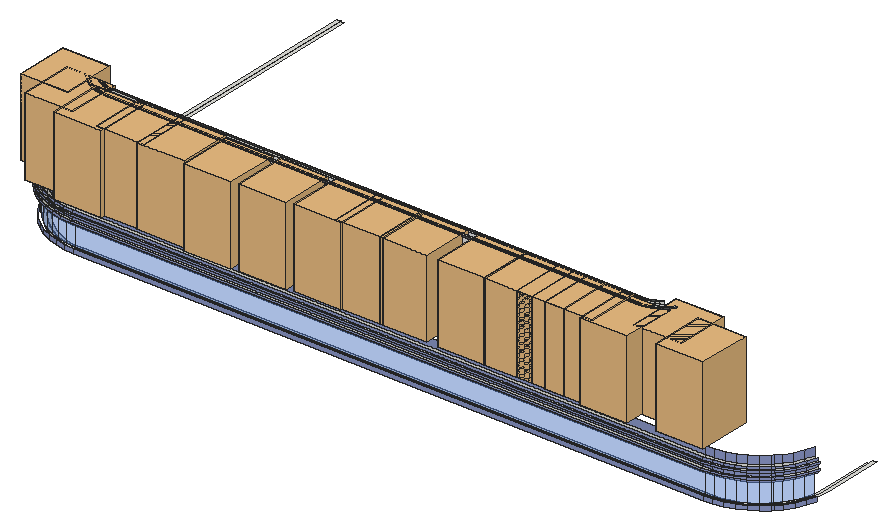
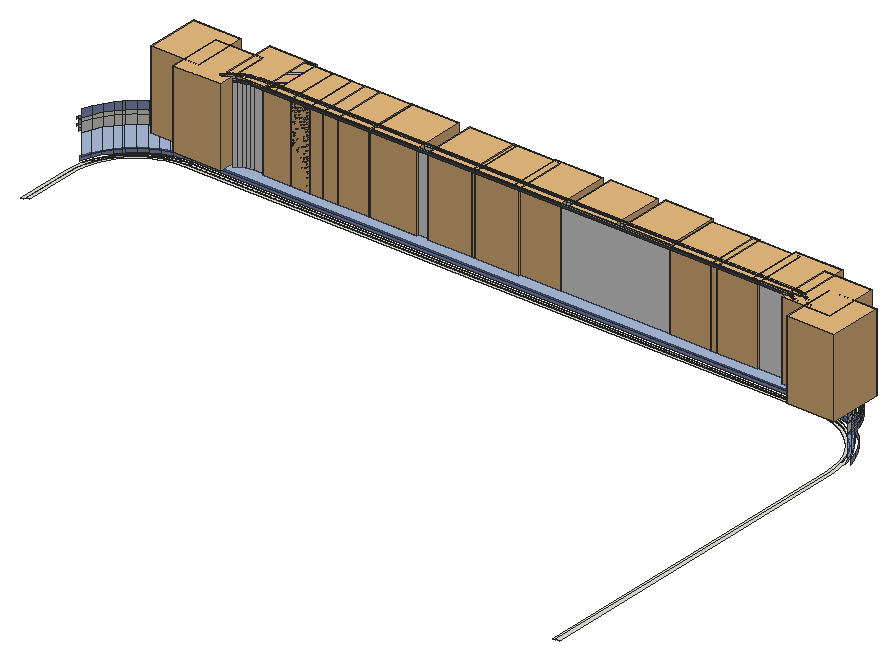
# SketchUp Ruby script. Lengths in inches.
U = 1.inch
M = Sketchup.active_model
def pt(a) = Geom::Point3d.new(a.map { |v| v * U })
def face(e, loops, mat)
  f = e.add_face(loops[0].map { |a| pt(a) })
  loops[1..].each { |l| e.add_face(l.map { |a| pt(a) }).erase! }
  f.material = f.back_material = mat if mat
  f
end
# faces: each face lists its corners as indices into pts; further lists are holes
def faces(e, pts, list, mat = nil) = list.each { |f| face(e, (f[0].is_a?(Array) ? f : [f]).map { |l| l.map { |i| pts[i] } }, mat) }
# xy, xz, yz: faces in a plane at the given z, y or x. An outline is a flat list of corners, or four numbers for a rectangle; further outlines are holes
def ring(l) = l.size == 4 ? [[l[0], l[1]], [l[2], l[1]], [l[2], l[3]], [l[0], l[3]]] : l.each_slice(2).to_a
def flat(e, list, mat, &to3) = list.each { |f| face(e, (f[0].is_a?(Array) ? f : [f]).map { |l| ring(l).map { |u, v| to3.(u, v) } }, mat) }
def xy(e, z, list, mat = nil) = flat(e, list, mat) { |x, y| [x, y, z] }
def xz(e, y, list, mat = nil) = flat(e, list, mat) { |x, z| [x, y, z] }
def yz(e, x, list, mat = nil) = flat(e, list, mat) { |y, z| [x, y, z] }
def lines(e, pts, list) = list.each { |a, b| e.add_line(pt(pts[a]), pt(pts[b])) }
# prism: a flat outline (further loops are holes) pulled along v
def prism(e, loops, v, mat = nil)
  f = face(e, loops, mat); d = Geom::Vector3d.new(v.map { |x| x * U })
  f.pushpull(f.normal.samedirection?(d) ? d.length : -d.length)
end
def box(e, o, s, mat = nil) = prism(e, [[o, [o[0] + s[0], o[1], o[2]], [o[0] + s[0], o[1] + s[1], o[2]], [o[0], o[1] + s[1], o[2]]]], [0, 0, s[2]], mat)
def at(x, y, z, deg = 0) = Geom::Transformation.translation(pt([x, y, z])) * Geom::Transformation.rotation(ORIGIN, Z_AXIS, deg.degrees)
def axes(o, x, y, z) = Geom::Transformation.new([*x, 0, *y, 0, *z, 0, *pt(o).to_a, 1])
def part(name) = M.definitions.add(name)
# library, detail: a bought-in or finely detailed component or shape, given as its bounding box
def library(name, o, s) = part(name).tap { |d| box(d.entities, o, s) }
def detail(e, o, s) = box(e.add_group.entities, o, s)
def put(e, d, t, mat = nil) = e.add_instance(d, t).tap { |i| i.material = mat if mat }
def group(e, t, mat = nil) = e.add_group.tap { |g| g.transformation = t; g.material = mat if mat }.entities
root = M.entities
M.materials.add("0326 AP 7207 CLASSIC PURPLE").color = [140, 152, 201]
M.materials.add("[Color M06]").color = [86, 86, 86]
M.materials.add("[Mirror 02]").color = [229, 229, 229]
M.materials.add("[Translucent Glass Blue]").color = [100, 149, 237]
M.materials["[Translucent Glass Blue]"].alpha = 0.5
c1 = library("Ficus elastica Belize 002",[-7.92,-8.8125,0.01],[22.14,24.73,36.43])
xy(root,252.375,[[45.79,28.41,41.61,28.68,37.51,29.49,33.55,30.84,29.8,32.6875,26.32,35.01,23.18,37.77,20.42,40.91,18.1,44.39,16.25,48.14,14.9,52.1,14.09,56.21,13.8125,60.38,13.8125,220.92,15.26,220.92,15.26,60.38,15.53,56.4,16.3,52.48,17.59,48.7,19.35,45.12,21.57,41.8,24.2,38.8,27.21,36.16,30.53,33.95,34.11,32.18,37.89,30.9,41.8,30.12,45.79,29.86,340.48,29.86,344.41,30.12,348.15,30.86,351.77,32.09,355.19,33.78,358.37,35.9,361.24,38.42,361.69,38.9375,363.76,41.29,365.88,44.46,367.57,47.89,368.8,51.51,369.54,55.25,369.8,59.18,369.8,84.09,371.25,84.09,371.25,59.13,370.98,55.0625,370.2,51.13,368.91,47.33,367.14,43.74,364.91,40.4,362.79,37.98,362.27,37.39,359.25,34.74,355.92,32.52,352.32,30.74,348.53,29.45,344.6,28.67,340.52,28.41]])
xy(root,252.5625,[[45.79,26.99,41.43,27.28,37.15,28.13,33.01,29.54,29.09,31.47,25.46,33.89,22.18,36.77,19.3,40.06,16.875,43.6875,14.94,47.6,13.54,51.74,12.6875,56.02,12.4,60.38,12.4,220.92,13.8125,220.92,13.8125,60.38,14.09,56.21,14.9,52.1,16.25,48.14,18.1,44.39,20.42,40.91,23.18,37.77,26.32,35.01,29.8,32.6875,33.55,30.84,37.51,29.49,41.61,28.68,45.79,28.41,340.52,28.41,344.6,28.67,348.53,29.45,352.32,30.74,355.92,32.52,359.25,34.74,362.27,37.39,362.79,37.98,364.91,40.4,367.14,43.74,368.91,47.33,370.2,51.13,370.98,55.0625,371.25,59.13,371.25,86.25,372.66,86.25,372.66,59.09,372.39,54.88,371.57,50.76,370.22,46.79,368.36,43.03,366.03,39.54,363.85,37.05,363.27,36.39,360.11,33.62,356.63,31.29,352.87,29.4375,348.89,28.09,344.78,27.27,340.57,26.99]])
xz(root,23.28,[[45.79,265.875,340.69,266.8125],[45.79,268.875,340.69,269.625]],"0326 AP 7207 CLASSIC PURPLE")
xz(root,24.43,[[45.79,265.875,340.65,266.8125],[45.79,268.875,340.65,269.625]])
xz(root,24.43,[[45.79,264.4375,340.65,265.875],[45.79,266.8125,340.65,268.875],[45.79,269.625,340.65,270.75]],"0326 AP 7207 CLASSIC PURPLE")
xz(root,24.97,[[45.79,252,340.64,254.0625]],"0326 AP 7207 CLASSIC PURPLE")
xz(root,26.25,[[45.79,264.4375,340.59,268.875],[45.79,268.875,340.59,270.75]])
xz(root,26.25,[[45.79,270.75,340.59,274.4375]],"0326 AP 7207 CLASSIC PURPLE")
xz(root,26.25,[[45.79,254.0625,340.59,264.4375]],"[Translucent Glass Blue]")
xz(root,26.99,[[45.79,252,340.57,252.5625]])
xz(root,28.41,[[45.79,252,340.52,252.375],[45.79,252.375,340.52,252.5625]])
xz(root,42.77,[[45.79,310.4375,294.9,311.125]],"[Color M06]")
xz(root,43.83,[[45.79,310.4375,294.87,311.125]])
xz(root,43.83,[[45.79,274.4375,294.87,310.4375]],"[Mirror 02]")
xz(root,47,[[45.79,310.4375,294.72,311.125]])
xz(root,47,[[45.79,274.4375,294.72,310.4375]],"[Mirror 02]")
xz(root,48.0625,[[45.79,310.4375,294.72,311.125]],"[Color M06]")
p = [[41.16,25.28,252],[45.79,24.97,252],[45.79,24.97,254.0625],[41.16,25.28,254.0625],[340.64,24.97,252],[345.04,25.26,252],
  [345.04,25.26,254.0625],[340.64,24.97,254.0625],[36.62,26.18,252],[36.62,26.18,254.0625],[349.42,26.13,252],[349.42,26.13,254.0625],
  [353.64,27.57,252],[353.64,27.57,254.0625],[32.24,27.67,252],[32.24,27.67,254.0625],[45.79,26.99,252],[41.43,27.28,252],
  [41.43,27.28,252.5625],[45.79,26.99,252.5625],[344.78,27.27,252],[340.57,26.99,252],[340.57,26.99,252.5625],[344.78,27.27,252.5625],
  [37.15,28.13,252],[37.15,28.13,252.5625],[348.89,28.09,252],[348.89,28.09,252.5625],[357.64,29.54,252],[357.64,29.54,254.0625],
  [28.08,29.72,252],[28.08,29.72,254.0625],[33.01,29.54,252],[33.01,29.54,252.5625],[352.87,29.4375,252],[352.87,29.4375,252.5625],
  [41.61,28.68,252],[45.79,28.41,252],[45.79,28.41,252.375],[41.61,28.68,252.375],[340.52,28.41,252],[344.6,28.67,252],
  [344.6,28.67,252.375],[340.52,28.41,252.375],[37.51,29.49,252],[37.51,29.49,252.375],[348.53,29.45,252],[348.53,29.45,252.375],
  [356.63,31.29,252],[356.63,31.29,252.5625],[29.09,31.47,252],[29.09,31.47,252.5625],[33.55,30.84,252],[33.55,30.84,252.375],
  [352.32,30.74,252],[352.32,30.74,252.375],[361.35,32.02,252],[361.35,32.02,254.0625],[24.23,32.29,252],[24.23,32.29,254.0625],
  [355.92,32.52,252],[355.92,32.52,252.375],[29.8,32.6875,252],[29.8,32.6875,252.375],[360.11,33.62,252],[360.11,33.62,252.5625],
  [25.46,33.89,252],[25.46,33.89,252.5625],[364.7,34.96,252],[364.7,34.96,254.0625],[20.75,35.34,252],[20.75,35.34,254.0625],
  [359.25,34.74,252],[359.25,34.74,252.375],[26.32,35.01,252],[26.32,35.01,252.375],[363.27,36.39,252],[363.27,36.39,252.5625],
  [22.18,36.77,252],[22.18,36.77,252.5625],[362.27,37.39,252],[362.27,37.39,252.375],[23.18,37.77,252],[23.18,37.77,252.375],
  [365.37,35.72,252],[365.37,35.72,254.0625],[17.7,38.83,252],[17.7,38.83,254.0625],[367.64,38.31,252],[367.64,38.31,254.0625],
  [363.85,37.05,252],[363.85,37.05,252.5625],[19.3,40.06,252],[19.3,40.06,252.5625],[366.03,39.54,252],[366.03,39.54,252.5625],
  [362.79,37.98,252],[362.79,37.98,252.375],[20.42,40.91,252],[20.42,40.91,252.375],[364.91,40.4,252],[364.91,40.4,252.375],
  [370.12,42.02,252],[370.12,42.02,254.0625],[15.125,42.68,252],[15.125,42.68,254.0625],[368.36,43.03,252],[368.36,43.03,252.5625],
  [16.875,43.6875,252],[16.875,43.6875,252.5625],[367.14,43.74,252],[367.14,43.74,252.375],[18.1,44.39,252],[18.1,44.39,252.375],
  [372.09,46.02,252],[372.09,46.02,254.0625],[13.08,46.83,252],[13.08,46.83,254.0625],[370.22,46.79,252],[370.22,46.79,252.5625],
  [14.94,47.6,252],[14.94,47.6,252.5625],[368.91,47.33,252],[368.91,47.33,252.375],[16.25,48.14,252],[16.25,48.14,252.375],
  [373.52,50.24,252],[373.52,50.24,254.0625],[11.59,51.22,252],[11.59,51.22,254.0625],[371.57,50.76,252],[371.57,50.76,252.5625],
  [370.2,51.13,252],[370.2,51.13,252.375],[13.54,51.74,252],[13.54,51.74,252.5625],[14.9,52.1,252],[14.9,52.1,252.375],
  [41.61,28.68,252.5625],[45.79,28.41,252.5625],[340.52,28.41,252.5625],[344.6,28.67,252.5625],[37.51,29.49,252.5625],[348.53,29.45,252.5625],
  [33.55,30.84,252.5625],[352.32,30.74,252.5625],[355.92,32.52,252.5625],[29.8,32.6875,252.5625],[359.25,34.74,252.5625],[26.32,35.01,252.5625],
  [362.27,37.39,252.5625],[23.18,37.77,252.5625],[362.79,37.98,252.5625],[20.42,40.91,252.5625],[364.91,40.4,252.5625],[367.14,43.74,252.5625],
  [18.1,44.39,252.5625],[368.91,47.33,252.5625],[16.25,48.14,252.5625],[370.2,51.13,252.5625],[14.9,52.1,252.5625],[45.79,26.25,254.0625],
  [45.79,26.25,264.4375],[41.33,26.54,264.4375],[41.33,26.54,254.0625],[344.88,26.53,254.0625],[344.88,26.53,264.4375],[340.59,26.25,264.4375],
  [340.59,26.25,254.0625],[36.95,27.41,264.4375],[36.95,27.41,254.0625],[349.09,27.37,254.0625],[349.09,27.37,264.4375],[32.73,28.85,264.4375],
  [32.73,28.85,254.0625],[353.15,28.75,254.0625],[353.15,28.75,264.4375],[357,30.65,254.0625],[357,30.65,264.4375],[28.72,30.82,264.4375],
  [28.72,30.82,254.0625],[360.57,33.03,254.0625],[360.57,33.03,264.4375],[25.01,33.3,264.4375],[25.01,33.3,254.0625],[363.8,35.86,254.0625],
  [363.8,35.86,264.4375],[21.65,36.25,264.4375],[21.65,36.25,254.0625],[364.41,36.56,254.0625],[364.41,36.56,264.4375],[18.71,39.6,264.4375],
  [18.71,39.6,254.0625],[366.625,39.09,254.0625],[366.625,39.09,264.4375],[369.01,42.66,254.0625],[369.01,42.66,264.4375],[16.23,43.31,264.4375],
  [16.23,43.31,254.0625],[370.91,46.51,254.0625],[370.91,46.51,264.4375],[14.25,47.32,264.4375],[14.25,47.32,254.0625],[372.29,50.57,254.0625],
  [372.29,50.57,264.4375],[12.82,51.55,264.4375],[12.82,51.55,254.0625],[45.79,24.43,265.875],[41.09,24.74,265.875],[41.09,24.74,264.4375],
  [45.79,24.43,264.4375],[345.11,24.73,265.875],[340.65,24.43,265.875],[340.65,24.43,264.4375],[345.11,24.73,264.4375],[36.48,25.66,265.875],
  [36.48,25.66,264.4375],[349.56,25.61,265.875],[349.56,25.61,264.4375],[353.85,27.07,265.875],[353.85,27.07,264.4375],[32.03,27.17,265.875],
  [32.03,27.17,264.4375],[45.79,26.25,268.875],[41.33,26.54,268.875],[344.88,26.53,268.875],[340.59,26.25,268.875],[36.95,27.41,268.875],
  [349.09,27.37,268.875],[357.91,29.07,265.875],[357.91,29.07,264.4375],[27.8125,29.25,265.875],[27.8125,29.25,264.4375],[32.73,28.85,268.875],
  [353.15,28.75,268.875],[357,30.65,268.875],[28.72,30.82,268.875],[361.68,31.59,265.875],[361.68,31.59,264.4375],[23.9,31.86,265.875],
  [23.9,31.86,264.4375],[360.57,33.03,268.875],[25.01,33.3,268.875],[365.08,34.57,265.875],[365.08,34.57,264.4375],[20.37,34.96,265.875],
  [20.37,34.96,264.4375],[363.8,35.86,268.875],[21.65,36.25,268.875],[365.77,35.36,265.875],[365.77,35.36,264.4375],[17.27,38.5,265.875],
  [17.27,38.5,264.4375],[368.07,37.98,265.875],[368.07,37.98,264.4375],[364.41,36.56,268.875],[18.71,39.6,268.875],[366.625,39.09,268.875],
  [370.59,41.75,265.875],[370.59,41.75,264.4375],[14.66,42.41,265.875],[14.66,42.41,264.4375],[369.01,42.66,268.875],[16.23,43.31,268.875],
  [372.59,45.81,265.875],[372.59,45.81,264.4375],[12.58,46.625,265.875],[12.58,46.625,264.4375],[370.91,46.51,268.875],[14.25,47.32,268.875],
  [374.05,50.1,265.875],[374.05,50.1,264.4375],[372.29,50.57,268.875],[11.07,51.08,265.875],[11.07,51.08,264.4375],[12.82,51.55,268.875],
  [40.94,23.6,265.875],[45.79,23.28,265.875],[45.79,23.28,266.8125],[40.94,23.6,266.8125],[340.69,23.28,265.875],[345.27,23.58,265.875],
  [345.27,23.58,266.8125],[340.69,23.28,266.8125],[36.18,24.54,265.875],[36.18,24.54,266.8125],[349.86,24.49,265.875],[349.86,24.49,266.8125],
  [45.79,24.43,266.8125],[41.09,24.74,266.8125],[345.11,24.73,266.8125],[340.65,24.43,266.8125],[31.59,26.1,265.875],[31.59,26.1,266.8125],
  [354.29,26,265.875],[354.29,26,266.8125],[36.48,25.66,266.8125],[349.56,25.61,266.8125],[353.85,27.07,266.8125],[32.03,27.17,266.8125],
  [358.49,28.07,265.875],[358.49,28.07,266.8125],[27.24,28.25,265.875],[27.24,28.25,266.8125],[357.91,29.07,266.8125],[27.8125,29.25,266.8125],
  [362.38,30.67,265.875],[362.38,30.67,266.8125],[23.2,30.95,265.875],[23.2,30.95,266.8125],[361.68,31.59,266.8125],[23.9,31.86,266.8125],
  [365.9,33.76,265.875],[365.9,33.76,266.8125],[19.55,34.15,265.875],[19.55,34.15,266.8125],[365.08,34.57,266.8125],[20.37,34.96,266.8125],
  [366.64,34.6,265.875],[366.64,34.6,266.8125],[16.35,37.8,265.875],[16.35,37.8,266.8125],[365.77,35.36,266.8125],[368.99,37.28,265.875],
  [368.99,37.28,266.8125],[17.27,38.5,266.8125],[368.07,37.98,266.8125],[371.59,41.17,265.875],[371.59,41.17,266.8125],[13.66,41.83,265.875],
  [13.66,41.83,266.8125],[370.59,41.75,266.8125],[14.66,42.41,266.8125],[373.66,45.37,265.875],[373.66,45.37,266.8125],[372.59,45.81,266.8125],
  [11.51,46.18,265.875],[11.51,46.18,266.8125],[12.58,46.625,266.8125],[375.16,49.8,265.875],[375.16,49.8,266.8125],[374.05,50.1,266.8125],
  [9.95,50.78,265.875],[9.95,50.78,266.8125],[11.07,51.08,266.8125],[41.09,24.74,268.875],[45.79,24.43,268.875],[340.65,24.43,268.875],
  [345.11,24.73,268.875],[36.48,25.66,268.875],[349.56,25.61,268.875],[353.85,27.07,268.875],[32.03,27.17,268.875],[357.91,29.07,268.875],
  [27.8125,29.25,268.875],[361.68,31.59,268.875],[23.9,31.86,268.875],[365.08,34.57,268.875],[20.37,34.96,268.875],[365.77,35.36,268.875],
  [17.27,38.5,268.875],[368.07,37.98,268.875],[370.59,41.75,268.875],[14.66,42.41,268.875],[372.59,45.81,268.875],[12.58,46.625,268.875],
  [374.05,50.1,268.875],[11.07,51.08,268.875],[40.94,23.6,268.875],[45.79,23.28,268.875],[45.79,23.28,269.625],[40.94,23.6,269.625],
  [340.69,23.28,268.875],[345.27,23.58,268.875],[345.27,23.58,269.625],[340.69,23.28,269.625],[36.18,24.55,268.875],[36.18,24.55,269.625],
  [349.86,24.5,268.875],[349.86,24.5,269.625],[45.79,24.43,269.625],[41.09,24.74,269.625],[345.11,24.73,269.625],[340.65,24.43,269.625],
  [31.59,26.11,268.875],[31.59,26.11,269.625],[354.29,26,268.875],[354.29,26,269.625],[36.48,25.66,269.625],[349.56,25.61,269.625],
  [353.85,27.07,269.625],[32.03,27.17,269.625],[358.49,28.07,268.875],[358.49,28.07,269.625],[27.24,28.25,268.875],[27.24,28.25,269.625],
  [45.79,26.25,270.75],[41.33,26.54,270.75],[344.88,26.53,270.75],[340.59,26.25,270.75],[36.95,27.41,270.75],[349.09,27.37,270.75],
  [357.91,29.07,269.625],[27.8125,29.25,269.625],[32.73,28.85,270.75],[353.15,28.75,270.75],[362.38,30.67,268.875],[362.38,30.67,269.625],
  [23.2,30.95,268.875],[23.2,30.95,269.625],[357,30.65,270.75],[28.72,30.82,270.75],[361.68,31.59,269.625],[23.9,31.86,269.625],
  [360.57,33.03,270.75],[365.9,33.76,268.875],[365.9,33.76,269.625],[25.01,33.3,270.75],[19.56,34.15,268.875],[19.56,34.15,269.625],
  [365.08,34.57,269.625],[20.37,34.96,269.625],[363.8,35.86,270.75],[21.65,36.25,270.75],[366.64,34.6,268.875],[366.64,34.6,269.625],
  [16.36,37.8,268.875],[16.36,37.8,269.625],[365.77,35.36,269.625],[368.98,37.28,268.875],[368.98,37.28,269.625],[17.27,38.5,269.625],
  [368.07,37.98,269.625],[364.41,36.56,270.75],[18.71,39.6,270.75],[366.625,39.09,270.75],[371.59,41.17,268.875],[371.59,41.17,269.625],
  [13.66,41.83,268.875],[13.66,41.83,269.625],[370.59,41.75,269.625],[14.66,42.41,269.625],[369.01,42.66,270.75],[16.23,43.31,270.75],
  [373.66,45.37,268.875],[373.66,45.37,269.625],[372.59,45.81,269.625],[11.51,46.18,268.875],[11.51,46.18,269.625],[12.58,46.625,269.625],
  [370.91,46.51,270.75],[14.25,47.32,270.75],[375.16,49.8,268.875],[375.16,49.8,269.625],[374.05,50.1,269.625],[9.95,50.78,268.875],
  [9.95,50.78,269.625],[372.29,50.57,270.75],[11.07,51.08,269.625],[12.82,51.55,270.75],[41.09,24.74,270.75],[45.79,24.43,270.75],
  [340.65,24.43,270.75],[345.11,24.73,270.75],[36.48,25.66,270.75],[349.56,25.61,270.75],[353.85,27.07,270.75],[32.03,27.17,270.75],
  [357.91,29.07,270.75],[27.8125,29.25,270.75],[361.68,31.59,270.75],[23.9,31.86,270.75],[365.08,34.57,270.75],[20.37,34.96,270.75],
  [365.77,35.36,270.75],[17.27,38.5,270.75],[368.07,37.98,270.75],[370.59,41.75,270.75],[14.66,42.41,270.75],[372.59,45.81,270.75],
  [12.58,46.625,270.75],[374.05,50.1,270.75],[11.07,51.08,270.75],[45.79,26.25,274.4375],[41.33,26.54,274.4375],[344.88,26.53,274.4375],
  [340.59,26.25,274.4375],[36.95,27.41,274.4375],[349.09,27.37,274.4375],[32.73,28.85,274.4375],[353.15,28.75,274.4375],[357,30.65,274.4375],
  [28.72,30.82,274.4375],[360.57,33.03,274.4375],[25.01,33.3,274.4375],[363.8,35.86,274.4375],[21.65,36.25,274.4375],[364.41,36.56,274.4375],
  [18.71,39.6,274.4375],[366.625,39.09,274.4375],[369.01,42.66,274.4375],[16.23,43.31,274.4375],[370.91,46.51,274.4375],[14.25,47.32,274.4375],
  [372.29,50.57,274.4375],[12.82,51.55,274.4375],[43.625,43.97,274.4375],[45.79,43.83,274.4375],[45.79,43.83,310.4375],[43.625,43.97,310.4375],
  [294.87,43.83,274.4375],[296.8,43.96,274.4375],[296.8,43.96,310.4375],[294.87,43.83,310.4375],[41.5,44.4,274.4375],[41.5,44.4,310.4375],
  [298.85,44.37,274.4375],[298.85,44.37,310.4375],[39.45,45.09,274.4375],[39.45,45.09,310.4375],[300.82,45.04,274.4375],[300.82,45.04,310.4375],
  [302.69,45.96,274.4375],[302.69,45.96,310.4375],[37.51,46.05,274.4375],[37.51,46.05,310.4375],[35.71,47.25,274.4375],[35.71,47.25,310.4375],
  [304.25,47,274.4375],[304.25,47,310.4375],[45.79,47,274.4375],[44.04,47.11,274.4375],[44.04,47.11,310.4375],[45.79,47,310.4375],
  [296.39,47.11,274.4375],[294.72,47,274.4375],[294.72,47,310.4375],[296.39,47.11,310.4375],[304.43,47.12,274.4375],[304.43,47.12,310.4375],
  [42.32,47.45,274.4375],[42.32,47.45,310.4375],[298.03,47.43,274.4375],[298.03,47.43,310.4375],[306,48.49,274.4375],[306,48.49,310.4375],
  [34.09,48.68,274.4375],[34.09,48.68,310.4375],[299.61,47.97,274.4375],[299.61,47.97,310.4375],[40.67,48.02,274.4375],[40.67,48.02,310.4375],
  [39.1,48.79,274.4375],[39.1,48.79,310.4375],[301.11,48.71,274.4375],[301.11,48.71,310.4375],[307.375,50.0625,274.4375],[307.375,50.0625,310.4375],
  [32.66,50.31,274.4375],[32.66,50.31,310.4375],[302.5,49.64,274.4375],[302.5,49.64,310.4375],[37.64,49.76,274.4375],[37.64,49.76,310.4375],
  [307.49,50.24,274.4375],[307.49,50.24,310.4375],[43.49,42.92,310.4375],[45.79,42.77,310.4375],[45.79,42.77,311.125],[43.49,42.92,311.125],
  [294.9,42.77,310.4375],[296.94,42.9,310.4375],[296.94,42.9,311.125],[294.9,42.77,311.125],[41.23,43.37,310.4375],[41.23,43.37,311.125],
  [299.125,43.34,310.4375],[299.125,43.34,311.125],[301.23,44.05,310.4375],[301.23,44.05,311.125],[39.05,44.11,310.4375],[39.05,44.11,311.125],
  [43.625,43.97,311.125],[45.79,43.83,311.125],[294.87,43.83,311.125],[296.8,43.96,311.125],[41.5,44.4,311.125],[298.85,44.37,311.125],
  [36.98,45.13,310.4375],[36.98,45.13,311.125],[303.23,45.04,310.4375],[303.23,45.04,311.125],[39.45,45.09,311.125],[300.82,45.04,311.125],
  [302.69,45.96,311.125],[304.84,46.11,310.4375],[304.84,46.11,311.125],[35.07,46.41,310.4375],[35.07,46.41,311.125],[37.51,46.05,311.125],
  [35.71,47.25,311.125],[304.25,47,311.125],[305.08,46.27,310.4375],[305.08,46.27,311.125],[306.75,47.74,310.4375],[306.75,47.74,311.125],
  [33.33,47.93,310.4375],[33.33,47.93,311.125],[45.79,47,311.125],[44.04,47.11,311.125],[296.39,47.11,311.125],[294.72,47,311.125],
  [304.43,47.12,311.125],[42.32,47.45,311.125],[298.03,47.43,311.125],[306,48.49,311.125],[34.09,48.68,311.125],[299.61,47.97,311.125],
  [40.67,48.02,311.125],[308.22,49.41,310.4375],[308.22,49.41,311.125],[31.81,49.66,310.4375],[31.81,49.66,311.125],[39.1,48.79,311.125],
  [301.11,48.71,311.125],[45.79,48.0625,310.4375],[44.18,48.17,310.4375],[44.18,48.17,311.125],[45.79,48.0625,311.125],[296.25,48.16,310.4375],
  [294.72,48.0625,310.4375],[294.72,48.0625,311.125],[296.25,48.16,311.125],[42.6,48.48,310.4375],[42.6,48.48,311.125],[297.75,48.46,310.4375],
  [297.75,48.46,311.125],[41.07,49,310.4375],[41.07,49,311.125],[299.2,48.95,310.4375],[299.2,48.95,311.125],[307.375,50.0625,311.125],
  [32.66,50.31,311.125],[302.5,49.64,311.125],[37.64,49.76,311.125],[39.63,49.71,310.4375],[39.63,49.71,311.125],[300.58,49.63,310.4375],
  [300.58,49.63,311.125],[308.375,49.65,310.4375],[308.375,49.65,311.125],[301.85,50.48,310.4375],[301.85,50.48,311.125],[45.79,29.86,252],
  [45.79,29.86,252.375],[340.48,29.86,252],[340.48,29.86,252.375],[364.41,36.56,252],[340.59,26.25,252],[45.79,26.25,252],
  [294.72,43.82,274.4375],[371.4,46.3,254.0625],[372.8,50.43,254.0625],[369.47,42.39,254.0625],[367.05,38.76,254.0625],[364.81,36.21,254.0625],
  [364.17,35.48,254.0625],[360.89,32.61,254.0625],[357.27,30.18,254.0625],[353.35,28.26,254.0625],[349.22,26.85,254.0625],[344.95,26,254.0625],
  [340.61,25.72,254.0625],[45.79,25.72,254.0625],[364.81,36.21,252],[340.61,25.72,252],[45.79,25.72,252]]
faces(root,p,[[0,1,2,3],[4,5,6,7],[8,0,3,9],[5,10,11,6],[10,12,13,11],[14,8,9,15],[12,28,29,13],[30,14,15,31],
  [28,56,57,29],[58,30,31,59],[56,68,69,57],[70,58,59,71],[68,84,85,69],[86,70,71,87],[84,88,89,85],[88,102,103,89],
  [104,86,87,105],[102,114,115,103],[116,104,105,117],[114,126,127,115],[128,116,117,129],[207,208,209,210],[211,212,213,214],[208,215,216,209],
  [217,211,214,218],[219,217,218,220],[215,221,222,216],[229,219,220,230],[221,231,232,222],[237,229,230,238],[231,239,240,232],[243,237,238,244],
  [239,245,246,240],[249,243,244,250],[245,251,252,246],[253,249,250,254],[258,253,254,259],[251,260,261,252],[264,258,259,265],[260,266,267,261],
  [270,264,265,271],[266,273,274,267],[276,277,278,279],[280,281,282,283],[284,276,279,285],[281,286,287,282],[292,284,285,293],[286,294,295,287],
  [294,300,301,295],[302,292,293,303],[300,306,307,301],[308,302,303,309],[306,312,313,307],[314,308,309,315],[312,318,319,313],[320,314,315,321],
  [318,323,324,319],[323,327,328,324],[329,320,321,330],[327,333,334,328],[336,329,330,337],[333,339,340,334],[342,336,337,343],[345,289,288,346],
  [347,291,290,348],[349,296,289,345],[348,290,297,350],[350,297,298,351],[352,299,296,349],[351,298,304,353],[354,305,299,352],[353,304,310,355],
  [356,311,305,354],[355,310,316,357],[358,317,311,356],[357,316,322,359],[360,325,317,358],[359,322,326,361],[361,326,331,362],[363,332,325,360],
  [362,331,335,364],[365,338,332,363],[364,335,341,366],[367,344,338,365],[368,369,370,371],[372,373,374,375],[376,368,371,377],[373,378,379,374],
  [384,376,377,385],[378,386,387,379],[386,392,393,387],[394,384,385,395],[392,406,407,393],[408,394,395,409],[406,415,416,407],[418,408,409,419],
  [415,424,425,416],[426,418,419,427],[424,429,430,425],[429,436,437,430],[438,426,427,439],[436,444,445,437],[447,438,439,448],[444,452,453,445],
  [455,447,448,456],[460,381,380,461],[462,383,382,463],[464,388,381,460],[463,382,389,465],[465,389,390,466],[467,391,388,464],[466,390,402,468],
  [469,403,391,467],[468,402,412,470],[471,413,403,469],[470,412,420,472],[473,421,413,471],[472,420,428,474],[475,431,421,473],[474,428,432,476],
  [476,432,440,477],[478,441,431,475],[477,440,446,479],[480,449,441,478],[479,446,454,481],[482,458,449,480],[483,484,397,396],[485,486,399,398],
  [484,487,400,397],[488,485,398,401],[487,489,404,400],[490,488,401,405],[491,490,405,410],[489,492,411,404],[493,491,410,414],[492,494,417,411],
  [495,493,414,422],[494,496,423,417],[497,495,422,433],[496,498,434,423],[499,497,433,435],[500,499,435,442],[498,501,443,434],[502,500,442,450],
  [501,503,451,443],[504,502,450,457],[503,505,459,451]],"0326 AP 7207 CLASSIC PURPLE")
faces(root,p,[[16,17,18,19],[20,21,22,23],[17,24,25,18],[26,20,23,27],[24,32,33,25],[34,26,27,35],[36,37,38,39],[40,41,42,43],
  [44,36,39,45],[41,46,47,42],[48,34,35,49],[32,50,51,33],[52,44,45,53],[46,54,55,47],[54,60,61,55],[62,52,53,63],
  [64,48,49,65],[50,66,67,51],[60,72,73,61],[74,62,63,75],[76,64,65,77],[66,78,79,67],[72,80,81,73],[82,74,75,83],
  [90,76,77,91],[78,92,93,79],[94,90,91,95],[80,96,97,81],[98,82,83,99],[96,100,101,97],[106,94,95,107],[92,108,109,93],
  [100,110,111,101],[112,98,99,113],[118,106,107,119],[108,120,121,109],[110,122,123,111],[124,112,113,125],[130,118,119,131],[122,132,133,123],
  [120,134,135,121],[136,124,125,137],[138,39,38,139],[140,43,42,141],[142,45,39,138],[141,42,47,143],[144,53,45,142],[143,47,55,145],
  [145,55,61,146],[147,63,53,144],[146,61,73,148],[149,75,63,147],[148,73,81,150],[151,83,75,149],[150,81,97,152],[153,99,83,151],
  [152,97,101,154],[154,101,111,155],[156,113,99,153],[155,111,123,157],[158,125,113,156],[157,123,133,159],[160,137,125,158],[162,223,224,163],
  [166,225,226,167],[163,224,227,169],[172,228,225,166],[169,227,233,173],[176,234,228,172],[178,235,234,176],[173,233,236,179],[182,241,235,178],
  [179,236,242,183],[186,247,241,182],[183,242,248,187],[190,255,247,186],[187,248,256,191],[194,257,255,190],[196,262,257,194],[191,256,263,197],
  [200,268,262,196],[197,263,269,201],[204,272,268,200],[201,269,275,205],[208,207,288,289],[212,211,290,291],[215,208,289,296],[211,217,297,290],
  [217,219,298,297],[221,215,296,299],[219,229,304,298],[231,221,299,305],[229,237,310,304],[239,231,305,311],[237,243,316,310],[245,239,311,317],
  [243,249,322,316],[251,245,317,325],[249,253,326,322],[253,258,331,326],[260,251,325,332],[258,264,335,331],[266,260,332,338],[264,270,341,335],
  [273,266,338,344],[345,346,380,381],[347,348,382,383],[349,345,381,388],[348,350,389,382],[350,351,390,389],[352,349,388,391],[224,223,396,397],
  [226,225,398,399],[227,224,397,400],[225,228,401,398],[351,353,402,390],[354,352,391,403],[233,227,400,404],[228,234,405,401],[234,235,410,405],
  [236,233,404,411],[353,355,412,402],[356,354,403,413],[235,241,414,410],[242,236,411,417],[355,357,420,412],[358,356,413,421],[241,247,422,414],
  [248,242,417,423],[357,359,428,420],[360,358,421,431],[359,361,432,428],[247,255,433,422],[256,248,423,434],[255,257,435,433],[361,362,440,432],
  [363,360,431,441],[257,262,442,435],[263,256,434,443],[362,364,446,440],[365,363,441,449],[262,268,450,442],[269,263,443,451],[364,366,454,446],
  [268,272,457,450],[367,365,449,458],[275,269,451,459],[508,509,582,583],[512,513,584,585],[509,515,586,582],[517,512,585,587],[515,519,592,586],
  [521,517,587,593],[523,521,593,594],[519,525,599,592],[525,527,600,599],[529,523,594,601],[532,533,608,609],[536,537,610,611],[539,529,601,612],
  [541,532,609,613],[537,543,614,610],[545,539,612,615],[527,547,616,600],[543,549,617,614],[551,541,613,618],[553,551,618,623],[549,555,624,617],
  [625,626,627,628],[626,633,634,627],[633,637,638,634],[557,545,615,641],[547,559,642,616],[555,561,643,624],[563,553,623,644],[637,645,646,638]])
faces(root,p,[[161,162,163,164],[165,166,167,168],[164,163,169,170],[171,172,166,165],[170,169,173,174],[175,176,172,171],[177,178,176,175],[174,173,179,180],
  [181,182,178,177],[180,179,183,184],[185,186,182,181],[184,183,187,188],[189,190,186,185],[188,187,191,192],[193,194,190,189],[195,196,194,193],
  [192,191,197,198],[199,200,196,195],[198,197,201,202],[203,204,200,199],[202,201,205,206]],"[Translucent Glass Blue]")
faces(root,p,[[506,507,508,509],[510,511,512,513],[514,506,509,515],[511,516,517,512],[518,514,515,519],[516,520,521,517],[520,522,523,521],[524,518,519,525],
  [526,524,525,527],[522,528,529,523],[530,531,532,533],[534,535,536,537],[528,538,539,529],[531,540,541,532],[542,534,537,543],[538,544,545,539],
  [546,526,527,547],[548,542,543,549],[540,550,551,541],[550,552,553,551],[554,548,549,555],[544,556,557,545],[558,546,547,559],[560,554,555,561],
  [552,562,563,553],[556,564,565,557]],"[Mirror 02]")
faces(root,p,[[566,567,568,569],[570,571,572,573],[574,566,569,575],[571,576,577,572],[576,578,579,577],[580,574,575,581],[588,580,581,589],[578,590,591,579],
  [590,595,596,591],[597,588,589,598],[595,602,603,596],[602,604,605,603],[606,597,598,607],[604,619,620,605],[621,606,607,622],[629,630,631,632],
  [635,629,632,636],[639,635,636,640],[647,639,640,648],[619,649,650,620],[651,647,648,652]],"[Color M06]")
lines(root,p,[[653,654],[655,656],[657,189],[658,168],[659,161],[660,510],[661,662],[663,661],[664,663],[665,664],[666,665],[667,666],
  [668,667],[669,668],[670,669],[671,670],[672,671],[673,672],[674,665],[675,672],[676,673]])
put(root,c1,at(108.36,29.76,274.4375))
put(root,c1,at(47.23,30.22,274.4375))
put(root,c1,at(133.47,30.5,274.4375))
put(root,c1,at(293.3,30.56,274.4375))
put(root,c1,at(158.78,31.32,274.4375))
put(root,c1,at(85.1,31.59,274.4375))
put(root,c1,at(275.78,31.91,274.4375))
put(root,c1,at(247.4375,31.91,274.4375))
put(root,c1,at(262.49,31.91,274.4375))
put(root,c1,at(225.7,31.91,274.4375))
put(root,c1,at(198.38,31.91,274.4375))
put(root,c1,at(177.75,31.91,274.4375))
put(root,c1,at(65.78,31.91,274.4375))
put(root,c1,at(327.17,32.78,274.4375))
put(root,c1,at(29.88,34.92,274.4375))
put(root,c1,at(311.87,39,274.4375))
put(root,c1,at(19.59,45.01,274.4375))
